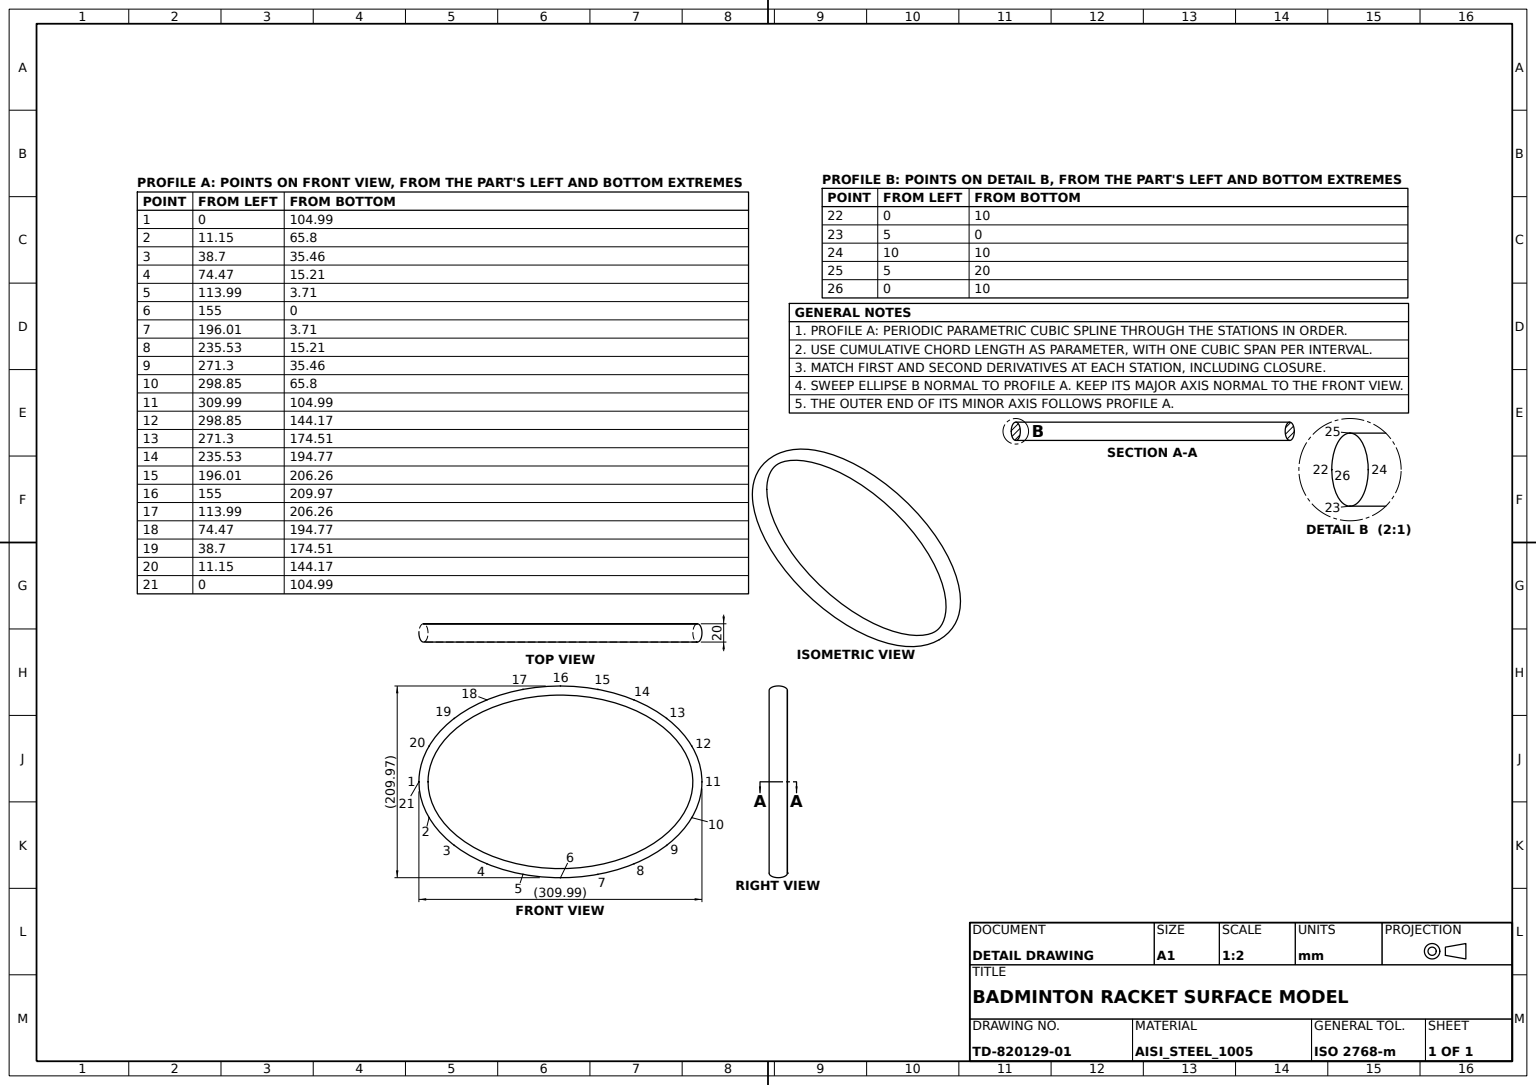
ISO-10303-21;
HEADER;
FILE_DESCRIPTION((''),'2;1');
FILE_NAME('','',(''),(''),'','','');
FILE_SCHEMA(('AUTOMOTIVE_DESIGN'));
ENDSEC;
DATA;
#1=APPLICATION_CONTEXT('');
#2=PRODUCT_CONTEXT('',#1,'mechanical');
#3=PRODUCT('','','',(#2));
#4=PRODUCT_DEFINITION_FORMATION('','',#3);
#5=PRODUCT_DEFINITION_CONTEXT('',#1,'design');
#6=PRODUCT_DEFINITION('','',#4,#5);
#7=PRODUCT_DEFINITION_SHAPE('','',#6);
#8=(LENGTH_UNIT()NAMED_UNIT(*)SI_UNIT(.MILLI.,.METRE.));
#9=(NAMED_UNIT(*)PLANE_ANGLE_UNIT()SI_UNIT($,.RADIAN.));
#10=(NAMED_UNIT(*)SI_UNIT($,.STERADIAN.)SOLID_ANGLE_UNIT());
#11=UNCERTAINTY_MEASURE_WITH_UNIT(LENGTH_MEASURE(0.005),#8,'distance_accuracy_value','');
#12=(GEOMETRIC_REPRESENTATION_CONTEXT(3)GLOBAL_UNCERTAINTY_ASSIGNED_CONTEXT((#11))GLOBAL_UNIT_ASSIGNED_CONTEXT((#8,#9,#10))REPRESENTATION_CONTEXT('',''));
#13=CARTESIAN_POINT('',(155.,0.,0.));
#14=VERTEX_POINT('',#13);
#15=VERTEX_LOOP('',#14);
#16=FACE_BOUND('',#15,.T.);
#17=CARTESIAN_POINT('',(155.,-4.365378,-3.535534));
#18=CARTESIAN_POINT('',(155.,4.365378,-3.535534));
#19=CARTESIAN_POINT('',(154.16152,13.313349,-3.535534));
#20=CARTESIAN_POINT('',(149.362746,30.331046,-3.535534));
#21=CARTESIAN_POINT('',(138.22226,49.513174,-3.535534));
#22=CARTESIAN_POINT('',(119.713466,67.928335,-3.535534));
#23=CARTESIAN_POINT('',(98.180606,82.120988,-3.535534));
#24=CARTESIAN_POINT('',(74.836894,92.619413,-3.535534));
#25=CARTESIAN_POINT('',(42.319091,102.226172,-3.535534));
#26=CARTESIAN_POINT('',(0.,106.826829,-3.535534));
#27=CARTESIAN_POINT('',(-42.31909,102.226172,-3.535534));
#28=CARTESIAN_POINT('',(-74.836894,92.619413,-3.535534));
#29=CARTESIAN_POINT('',(-98.180606,82.120988,-3.535534));
#30=CARTESIAN_POINT('',(-119.713466,67.928335,-3.535534));
#31=CARTESIAN_POINT('',(-138.22226,49.513174,-3.535534));
#32=CARTESIAN_POINT('',(-149.362746,30.331046,-3.535534));
#33=CARTESIAN_POINT('',(-154.161522,13.313342,-3.535534));
#34=CARTESIAN_POINT('',(-155.409023,0.000001,-3.535534));
#35=CARTESIAN_POINT('',(-154.161522,-13.313345,-3.535534));
#36=CARTESIAN_POINT('',(-149.362746,-30.331043,-3.535534));
#37=CARTESIAN_POINT('',(-138.22226,-49.513175,-3.535534));
#38=CARTESIAN_POINT('',(-119.713466,-67.928335,-3.535534));
#39=CARTESIAN_POINT('',(-98.180606,-82.120988,-3.535534));
#40=CARTESIAN_POINT('',(-74.836894,-92.619413,-3.535534));
#41=CARTESIAN_POINT('',(-42.319091,-102.226172,-3.535534));
#42=CARTESIAN_POINT('',(-0.000001,-106.82683,-3.535534));
#43=CARTESIAN_POINT('',(42.319096,-102.226171,-3.535534));
#44=CARTESIAN_POINT('',(74.836893,-92.619413,-3.535534));
#45=CARTESIAN_POINT('',(98.180607,-82.120988,-3.535534));
#46=CARTESIAN_POINT('',(119.713466,-67.928335,-3.535534));
#47=CARTESIAN_POINT('',(138.22226,-49.513174,-3.535534));
#48=CARTESIAN_POINT('',(149.362746,-30.331046,-3.535534));
#49=CARTESIAN_POINT('',(154.16152,-13.313349,-3.535534));
#50=CARTESIAN_POINT('',(155.,-4.365378,3.535534));
#51=CARTESIAN_POINT('',(155.,4.365378,3.535534));
#52=CARTESIAN_POINT('',(154.16152,13.313349,3.535534));
#53=CARTESIAN_POINT('',(149.362746,30.331046,3.535534));
#54=CARTESIAN_POINT('',(138.22226,49.513174,3.535534));
#55=CARTESIAN_POINT('',(119.713466,67.928335,3.535534));
#56=CARTESIAN_POINT('',(98.180606,82.120988,3.535534));
#57=CARTESIAN_POINT('',(74.836894,92.619413,3.535534));
#58=CARTESIAN_POINT('',(42.319091,102.226172,3.535534));
#59=CARTESIAN_POINT('',(0.,106.826829,3.535534));
#60=CARTESIAN_POINT('',(-42.31909,102.226172,3.535534));
#61=CARTESIAN_POINT('',(-74.836894,92.619413,3.535534));
#62=CARTESIAN_POINT('',(-98.180606,82.120988,3.535534));
#63=CARTESIAN_POINT('',(-119.713466,67.928335,3.535534));
#64=CARTESIAN_POINT('',(-138.22226,49.513174,3.535534));
#65=CARTESIAN_POINT('',(-149.362746,30.331046,3.535534));
#66=CARTESIAN_POINT('',(-154.161522,13.313342,3.535534));
#67=CARTESIAN_POINT('',(-155.409023,0.000001,3.535534));
#68=CARTESIAN_POINT('',(-154.161522,-13.313345,3.535534));
#69=CARTESIAN_POINT('',(-149.362746,-30.331043,3.535534));
#70=CARTESIAN_POINT('',(-138.22226,-49.513175,3.535534));
#71=CARTESIAN_POINT('',(-119.713466,-67.928335,3.535534));
#72=CARTESIAN_POINT('',(-98.180606,-82.120988,3.535534));
#73=CARTESIAN_POINT('',(-74.836894,-92.619413,3.535534));
#74=CARTESIAN_POINT('',(-42.319091,-102.226172,3.535534));
#75=CARTESIAN_POINT('',(-0.000001,-106.82683,3.535534));
#76=CARTESIAN_POINT('',(42.319096,-102.226171,3.535534));
#77=CARTESIAN_POINT('',(74.836893,-92.619413,3.535534));
#78=CARTESIAN_POINT('',(98.180607,-82.120988,3.535534));
#79=CARTESIAN_POINT('',(119.713466,-67.928335,3.535534));
#80=CARTESIAN_POINT('',(138.22226,-49.513174,3.535534));
#81=CARTESIAN_POINT('',(149.362746,-30.331046,3.535534));
#82=CARTESIAN_POINT('',(154.16152,-13.313349,3.535534));
#83=CARTESIAN_POINT('',(154.116117,-4.324056,8.232233));
#84=CARTESIAN_POINT('',(154.116117,4.324056,8.232233));
#85=CARTESIAN_POINT('',(153.288993,13.150839,8.232233));
#86=CARTESIAN_POINT('',(148.542341,29.983695,8.232233));
#87=CARTESIAN_POINT('',(137.516365,48.968656,8.232233));
#88=CARTESIAN_POINT('',(119.152954,67.239169,8.232233));
#89=CARTESIAN_POINT('',(97.753393,81.343963,8.232233));
#90=CARTESIAN_POINT('',(74.529005,91.788724,8.232233));
#91=CARTESIAN_POINT('',(42.144722,101.356037,8.232233));
#92=CARTESIAN_POINT('',(0.,105.937738,8.232233));
#93=CARTESIAN_POINT('',(-42.144721,101.356037,8.232233));
#94=CARTESIAN_POINT('',(-74.529005,91.788723,8.232233));
#95=CARTESIAN_POINT('',(-97.753393,81.343963,8.232233));
#96=CARTESIAN_POINT('',(-119.152954,67.239169,8.232233));
#97=CARTESIAN_POINT('',(-137.516365,48.968656,8.232233));
#98=CARTESIAN_POINT('',(-148.542341,29.983695,8.232233));
#99=CARTESIAN_POINT('',(-153.288994,13.150833,8.232233));
#100=CARTESIAN_POINT('',(-154.521268,0.000001,8.232233));
#101=CARTESIAN_POINT('',(-153.288994,-13.150836,8.232233));
#102=CARTESIAN_POINT('',(-148.542342,-29.983692,8.232233));
#103=CARTESIAN_POINT('',(-137.516364,-48.968657,8.232233));
#104=CARTESIAN_POINT('',(-119.152954,-67.239169,8.232233));
#105=CARTESIAN_POINT('',(-97.753393,-81.343963,8.232233));
#106=CARTESIAN_POINT('',(-74.529005,-91.788724,8.232233));
#107=CARTESIAN_POINT('',(-42.144722,-101.356037,8.232233));
#108=CARTESIAN_POINT('',(-0.000001,-105.937739,8.232233));
#109=CARTESIAN_POINT('',(42.144726,-101.356036,8.232233));
#110=CARTESIAN_POINT('',(74.529004,-91.788724,8.232233));
#111=CARTESIAN_POINT('',(97.753393,-81.343963,8.232233));
#112=CARTESIAN_POINT('',(119.152954,-67.239169,8.232233));
#113=CARTESIAN_POINT('',(137.516365,-48.968656,8.232233));
#114=CARTESIAN_POINT('',(148.542341,-29.983695,8.232233));
#115=CARTESIAN_POINT('',(153.288993,-13.150839,8.232233));
#116=CARTESIAN_POINT('',(151.767767,-4.214269,10.));
#117=CARTESIAN_POINT('',(151.767767,4.214269,10.));
#118=CARTESIAN_POINT('',(150.970814,12.719074,10.));
#119=CARTESIAN_POINT('',(146.362646,29.060832,10.));
#120=CARTESIAN_POINT('',(135.640904,47.521951,10.));
#121=CARTESIAN_POINT('',(117.663756,65.408156,10.));
#122=CARTESIAN_POINT('',(96.61835,79.27952,10.));
#123=CARTESIAN_POINT('',(73.710988,89.581704,10.));
#124=CARTESIAN_POINT('',(41.681448,99.044215,10.));
#125=CARTESIAN_POINT('',(0.,103.575552,10.));
#126=CARTESIAN_POINT('',(-41.681447,99.044216,10.));
#127=CARTESIAN_POINT('',(-73.710988,89.581704,10.));
#128=CARTESIAN_POINT('',(-96.61835,79.27952,10.));
#129=CARTESIAN_POINT('',(-117.663756,65.408156,10.));
#130=CARTESIAN_POINT('',(-135.640904,47.521951,10.));
#131=CARTESIAN_POINT('',(-146.362646,29.060832,10.));
#132=CARTESIAN_POINT('',(-150.970815,12.719071,10.));
#133=CARTESIAN_POINT('',(-152.162631,0.000001,10.));
#134=CARTESIAN_POINT('',(-150.970814,-12.719075,10.));
#135=CARTESIAN_POINT('',(-146.362647,-29.060829,10.));
#136=CARTESIAN_POINT('',(-135.640904,-47.521952,10.));
#137=CARTESIAN_POINT('',(-117.663756,-65.408156,10.));
#138=CARTESIAN_POINT('',(-96.61835,-79.27952,10.));
#139=CARTESIAN_POINT('',(-73.710988,-89.581704,10.));
#140=CARTESIAN_POINT('',(-41.681448,-99.044215,10.));
#141=CARTESIAN_POINT('',(-0.000001,-103.575553,10.));
#142=CARTESIAN_POINT('',(41.681452,-99.044214,10.));
#143=CARTESIAN_POINT('',(73.710987,-89.581704,10.));
#144=CARTESIAN_POINT('',(96.618351,-79.27952,10.));
#145=CARTESIAN_POINT('',(117.663756,-65.408156,10.));
#146=CARTESIAN_POINT('',(135.640904,-47.521951,10.));
#147=CARTESIAN_POINT('',(146.362646,-29.060832,10.));
#148=CARTESIAN_POINT('',(150.970814,-12.719074,10.));
#149=CARTESIAN_POINT('',(148.232233,-4.048981,10.));
#150=CARTESIAN_POINT('',(148.232233,4.048981,10.));
#151=CARTESIAN_POINT('',(147.480705,12.069035,10.));
#152=CARTESIAN_POINT('',(143.081029,27.671426,10.));
#153=CARTESIAN_POINT('',(132.817323,45.343879,10.));
#154=CARTESIAN_POINT('',(115.421709,62.651492,10.));
#155=CARTESIAN_POINT('',(94.909498,76.171419,10.));
#156=CARTESIAN_POINT('',(72.479431,86.258947,10.));
#157=CARTESIAN_POINT('',(40.98397,95.563675,10.));
#158=CARTESIAN_POINT('',(0.,100.019187,10.));
#159=CARTESIAN_POINT('',(-40.983969,95.563676,10.));
#160=CARTESIAN_POINT('',(-72.479431,86.258947,10.));
#161=CARTESIAN_POINT('',(-94.909498,76.171419,10.));
#162=CARTESIAN_POINT('',(-115.421709,62.651492,10.));
#163=CARTESIAN_POINT('',(-132.817323,45.343879,10.));
#164=CARTESIAN_POINT('',(-143.081029,27.671426,10.));
#165=CARTESIAN_POINT('',(-147.480704,12.069037,10.));
#166=CARTESIAN_POINT('',(-148.61161,0.000001,10.));
#167=CARTESIAN_POINT('',(-147.480703,-12.06904,10.));
#168=CARTESIAN_POINT('',(-143.081029,-27.671423,10.));
#169=CARTESIAN_POINT('',(-132.817322,-45.34388,10.));
#170=CARTESIAN_POINT('',(-115.421709,-62.651492,10.));
#171=CARTESIAN_POINT('',(-94.909498,-76.171419,10.));
#172=CARTESIAN_POINT('',(-72.479431,-86.258947,10.));
#173=CARTESIAN_POINT('',(-40.98397,-95.563675,10.));
#174=CARTESIAN_POINT('',(-0.000001,-100.019188,10.));
#175=CARTESIAN_POINT('',(40.983974,-95.563674,10.));
#176=CARTESIAN_POINT('',(72.47943,-86.258948,10.));
#177=CARTESIAN_POINT('',(94.909498,-76.171419,10.));
#178=CARTESIAN_POINT('',(115.421709,-62.651492,10.));
#179=CARTESIAN_POINT('',(132.817323,-45.343879,10.));
#180=CARTESIAN_POINT('',(143.081029,-27.671426,10.));
#181=CARTESIAN_POINT('',(147.480705,-12.069035,10.));
#182=CARTESIAN_POINT('',(145.883883,-3.939194,8.232233));
#183=CARTESIAN_POINT('',(145.883883,3.939194,8.232233));
#184=CARTESIAN_POINT('',(145.162526,11.63727,8.232233));
#185=CARTESIAN_POINT('',(140.901334,26.748563,8.232233));
#186=CARTESIAN_POINT('',(130.941862,43.897174,8.232233));
#187=CARTESIAN_POINT('',(113.932511,60.820478,8.232233));
#188=CARTESIAN_POINT('',(93.774455,74.106976,8.232233));
#189=CARTESIAN_POINT('',(71.661415,84.051927,8.232233));
#190=CARTESIAN_POINT('',(40.520696,93.251854,8.232233));
#191=CARTESIAN_POINT('',(0.,97.657001,8.232233));
#192=CARTESIAN_POINT('',(-40.520695,93.251854,8.232233));
#193=CARTESIAN_POINT('',(-71.661415,84.051927,8.232233));
#194=CARTESIAN_POINT('',(-93.774455,74.106976,8.232233));
#195=CARTESIAN_POINT('',(-113.932511,60.820478,8.232233));
#196=CARTESIAN_POINT('',(-130.941862,43.897174,8.232233));
#197=CARTESIAN_POINT('',(-140.901334,26.748563,8.232233));
#198=CARTESIAN_POINT('',(-145.162525,11.637276,8.232233));
#199=CARTESIAN_POINT('',(-146.252973,0.000001,8.232233));
#200=CARTESIAN_POINT('',(-145.162524,-11.637279,8.232233));
#201=CARTESIAN_POINT('',(-140.901334,-26.74856,8.232233));
#202=CARTESIAN_POINT('',(-130.941862,-43.897175,8.232233));
#203=CARTESIAN_POINT('',(-113.932511,-60.820478,8.232233));
#204=CARTESIAN_POINT('',(-93.774455,-74.106976,8.232233));
#205=CARTESIAN_POINT('',(-71.661415,-84.051927,8.232233));
#206=CARTESIAN_POINT('',(-40.520696,-93.251854,8.232233));
#207=CARTESIAN_POINT('',(-0.000001,-97.657002,8.232233));
#208=CARTESIAN_POINT('',(40.5207,-93.251853,8.232233));
#209=CARTESIAN_POINT('',(71.661413,-84.051928,8.232233));
#210=CARTESIAN_POINT('',(93.774455,-74.106976,8.232233));
#211=CARTESIAN_POINT('',(113.932511,-60.820478,8.232233));
#212=CARTESIAN_POINT('',(130.941862,-43.897174,8.232233));
#213=CARTESIAN_POINT('',(140.901334,-26.748563,8.232233));
#214=CARTESIAN_POINT('',(145.162526,-11.637269,8.232233));
#215=CARTESIAN_POINT('',(145.,-3.897872,3.535534));
#216=CARTESIAN_POINT('',(145.,3.897872,3.535534));
#217=CARTESIAN_POINT('',(144.289999,11.47476,3.535534));
#218=CARTESIAN_POINT('',(140.080929,26.401211,3.535534));
#219=CARTESIAN_POINT('',(130.235967,43.352656,3.535534));
#220=CARTESIAN_POINT('',(113.371999,60.131312,3.535534));
#221=CARTESIAN_POINT('',(93.347242,73.329951,3.535534));
#222=CARTESIAN_POINT('',(71.353525,83.221238,3.535534));
#223=CARTESIAN_POINT('',(40.346327,92.381719,3.535534));
#224=CARTESIAN_POINT('',(0.,96.76791,3.535534));
#225=CARTESIAN_POINT('',(-40.346326,92.381719,3.535534));
#226=CARTESIAN_POINT('',(-71.353525,83.221238,3.535534));
#227=CARTESIAN_POINT('',(-93.347242,73.329951,3.535534));
#228=CARTESIAN_POINT('',(-113.371999,60.131312,3.535534));
#229=CARTESIAN_POINT('',(-130.235967,43.352656,3.535534));
#230=CARTESIAN_POINT('',(-140.080929,26.401211,3.535534));
#231=CARTESIAN_POINT('',(-144.289997,11.474767,3.535534));
#232=CARTESIAN_POINT('',(-145.365218,0.000001,3.535534));
#233=CARTESIAN_POINT('',(-144.289996,-11.47477,3.535534));
#234=CARTESIAN_POINT('',(-140.08093,-26.401209,3.535534));
#235=CARTESIAN_POINT('',(-130.235966,-43.352657,3.535534));
#236=CARTESIAN_POINT('',(-113.371999,-60.131312,3.535534));
#237=CARTESIAN_POINT('',(-93.347242,-73.329951,3.535534));
#238=CARTESIAN_POINT('',(-71.353525,-83.221238,3.535534));
#239=CARTESIAN_POINT('',(-40.346327,-92.381719,3.535534));
#240=CARTESIAN_POINT('',(-0.000001,-96.76791,3.535534));
#241=CARTESIAN_POINT('',(40.346331,-92.381718,3.535534));
#242=CARTESIAN_POINT('',(71.353524,-83.221239,3.535534));
#243=CARTESIAN_POINT('',(93.347242,-73.329951,3.535534));
#244=CARTESIAN_POINT('',(113.371999,-60.131312,3.535534));
#245=CARTESIAN_POINT('',(130.235967,-43.352656,3.535534));
#246=CARTESIAN_POINT('',(140.080929,-26.401211,3.535534));
#247=CARTESIAN_POINT('',(144.289999,-11.47476,3.535534));
#248=CARTESIAN_POINT('',(145.,-3.897872,-3.535534));
#249=CARTESIAN_POINT('',(145.,3.897872,-3.535534));
#250=CARTESIAN_POINT('',(144.289999,11.47476,-3.535534));
#251=CARTESIAN_POINT('',(140.080929,26.401211,-3.535534));
#252=CARTESIAN_POINT('',(130.235967,43.352656,-3.535534));
#253=CARTESIAN_POINT('',(113.371999,60.131312,-3.535534));
#254=CARTESIAN_POINT('',(93.347242,73.329951,-3.535534));
#255=CARTESIAN_POINT('',(71.353525,83.221238,-3.535534));
#256=CARTESIAN_POINT('',(40.346327,92.381719,-3.535534));
#257=CARTESIAN_POINT('',(0.,96.76791,-3.535534));
#258=CARTESIAN_POINT('',(-40.346326,92.381719,-3.535534));
#259=CARTESIAN_POINT('',(-71.353525,83.221238,-3.535534));
#260=CARTESIAN_POINT('',(-93.347242,73.329951,-3.535534));
#261=CARTESIAN_POINT('',(-113.371999,60.131312,-3.535534));
#262=CARTESIAN_POINT('',(-130.235967,43.352656,-3.535534));
#263=CARTESIAN_POINT('',(-140.080929,26.401211,-3.535534));
#264=CARTESIAN_POINT('',(-144.289997,11.474767,-3.535534));
#265=CARTESIAN_POINT('',(-145.365218,0.000001,-3.535534));
#266=CARTESIAN_POINT('',(-144.289996,-11.47477,-3.535534));
#267=CARTESIAN_POINT('',(-140.08093,-26.401209,-3.535534));
#268=CARTESIAN_POINT('',(-130.235966,-43.352657,-3.535534));
#269=CARTESIAN_POINT('',(-113.371999,-60.131312,-3.535534));
#270=CARTESIAN_POINT('',(-93.347242,-73.329951,-3.535534));
#271=CARTESIAN_POINT('',(-71.353525,-83.221238,-3.535534));
#272=CARTESIAN_POINT('',(-40.346327,-92.381719,-3.535534));
#273=CARTESIAN_POINT('',(-0.000001,-96.76791,-3.535534));
#274=CARTESIAN_POINT('',(40.346331,-92.381718,-3.535534));
#275=CARTESIAN_POINT('',(71.353524,-83.221239,-3.535534));
#276=CARTESIAN_POINT('',(93.347242,-73.329951,-3.535534));
#277=CARTESIAN_POINT('',(113.371999,-60.131312,-3.535534));
#278=CARTESIAN_POINT('',(130.235967,-43.352656,-3.535534));
#279=CARTESIAN_POINT('',(140.080929,-26.401211,-3.535534));
#280=CARTESIAN_POINT('',(144.289999,-11.47476,-3.535534));
#281=CARTESIAN_POINT('',(145.883883,-3.939194,-8.232233));
#282=CARTESIAN_POINT('',(145.883883,3.939194,-8.232233));
#283=CARTESIAN_POINT('',(145.162526,11.63727,-8.232233));
#284=CARTESIAN_POINT('',(140.901334,26.748563,-8.232233));
#285=CARTESIAN_POINT('',(130.941862,43.897174,-8.232233));
#286=CARTESIAN_POINT('',(113.932511,60.820478,-8.232233));
#287=CARTESIAN_POINT('',(93.774455,74.106976,-8.232233));
#288=CARTESIAN_POINT('',(71.661415,84.051927,-8.232233));
#289=CARTESIAN_POINT('',(40.520696,93.251854,-8.232233));
#290=CARTESIAN_POINT('',(0.,97.657001,-8.232233));
#291=CARTESIAN_POINT('',(-40.520695,93.251854,-8.232233));
#292=CARTESIAN_POINT('',(-71.661415,84.051927,-8.232233));
#293=CARTESIAN_POINT('',(-93.774455,74.106976,-8.232233));
#294=CARTESIAN_POINT('',(-113.932511,60.820478,-8.232233));
#295=CARTESIAN_POINT('',(-130.941862,43.897174,-8.232233));
#296=CARTESIAN_POINT('',(-140.901334,26.748563,-8.232233));
#297=CARTESIAN_POINT('',(-145.162525,11.637276,-8.232233));
#298=CARTESIAN_POINT('',(-146.252973,0.000001,-8.232233));
#299=CARTESIAN_POINT('',(-145.162524,-11.637279,-8.232233));
#300=CARTESIAN_POINT('',(-140.901334,-26.74856,-8.232233));
#301=CARTESIAN_POINT('',(-130.941862,-43.897175,-8.232233));
#302=CARTESIAN_POINT('',(-113.932511,-60.820478,-8.232233));
#303=CARTESIAN_POINT('',(-93.774455,-74.106976,-8.232233));
#304=CARTESIAN_POINT('',(-71.661415,-84.051927,-8.232233));
#305=CARTESIAN_POINT('',(-40.520696,-93.251854,-8.232233));
#306=CARTESIAN_POINT('',(-0.000001,-97.657002,-8.232233));
#307=CARTESIAN_POINT('',(40.5207,-93.251853,-8.232233));
#308=CARTESIAN_POINT('',(71.661413,-84.051928,-8.232233));
#309=CARTESIAN_POINT('',(93.774455,-74.106976,-8.232233));
#310=CARTESIAN_POINT('',(113.932511,-60.820478,-8.232233));
#311=CARTESIAN_POINT('',(130.941862,-43.897174,-8.232233));
#312=CARTESIAN_POINT('',(140.901334,-26.748563,-8.232233));
#313=CARTESIAN_POINT('',(145.162526,-11.637269,-8.232233));
#314=CARTESIAN_POINT('',(148.232233,-4.048981,-10.));
#315=CARTESIAN_POINT('',(148.232233,4.048981,-10.));
#316=CARTESIAN_POINT('',(147.480705,12.069035,-10.));
#317=CARTESIAN_POINT('',(143.081029,27.671426,-10.));
#318=CARTESIAN_POINT('',(132.817323,45.343879,-10.));
#319=CARTESIAN_POINT('',(115.421709,62.651492,-10.));
#320=CARTESIAN_POINT('',(94.909498,76.171419,-10.));
#321=CARTESIAN_POINT('',(72.479431,86.258947,-10.));
#322=CARTESIAN_POINT('',(40.98397,95.563675,-10.));
#323=CARTESIAN_POINT('',(0.,100.019187,-10.));
#324=CARTESIAN_POINT('',(-40.983969,95.563676,-10.));
#325=CARTESIAN_POINT('',(-72.479431,86.258947,-10.));
#326=CARTESIAN_POINT('',(-94.909498,76.171419,-10.));
#327=CARTESIAN_POINT('',(-115.421709,62.651492,-10.));
#328=CARTESIAN_POINT('',(-132.817323,45.343879,-10.));
#329=CARTESIAN_POINT('',(-143.081029,27.671426,-10.));
#330=CARTESIAN_POINT('',(-147.480704,12.069037,-10.));
#331=CARTESIAN_POINT('',(-148.61161,0.000001,-10.));
#332=CARTESIAN_POINT('',(-147.480703,-12.06904,-10.));
#333=CARTESIAN_POINT('',(-143.081029,-27.671423,-10.));
#334=CARTESIAN_POINT('',(-132.817322,-45.34388,-10.));
#335=CARTESIAN_POINT('',(-115.421709,-62.651492,-10.));
#336=CARTESIAN_POINT('',(-94.909498,-76.171419,-10.));
#337=CARTESIAN_POINT('',(-72.479431,-86.258947,-10.));
#338=CARTESIAN_POINT('',(-40.98397,-95.563675,-10.));
#339=CARTESIAN_POINT('',(-0.000001,-100.019188,-10.));
#340=CARTESIAN_POINT('',(40.983974,-95.563674,-10.));
#341=CARTESIAN_POINT('',(72.47943,-86.258948,-10.));
#342=CARTESIAN_POINT('',(94.909498,-76.171419,-10.));
#343=CARTESIAN_POINT('',(115.421709,-62.651492,-10.));
#344=CARTESIAN_POINT('',(132.817323,-45.343879,-10.));
#345=CARTESIAN_POINT('',(143.081029,-27.671426,-10.));
#346=CARTESIAN_POINT('',(147.480705,-12.069035,-10.));
#347=CARTESIAN_POINT('',(151.767767,-4.214269,-10.));
#348=CARTESIAN_POINT('',(151.767767,4.214269,-10.));
#349=CARTESIAN_POINT('',(150.970814,12.719074,-10.));
#350=CARTESIAN_POINT('',(146.362646,29.060832,-10.));
#351=CARTESIAN_POINT('',(135.640904,47.521951,-10.));
#352=CARTESIAN_POINT('',(117.663756,65.408156,-10.));
#353=CARTESIAN_POINT('',(96.61835,79.27952,-10.));
#354=CARTESIAN_POINT('',(73.710988,89.581704,-10.));
#355=CARTESIAN_POINT('',(41.681448,99.044215,-10.));
#356=CARTESIAN_POINT('',(0.,103.575552,-10.));
#357=CARTESIAN_POINT('',(-41.681447,99.044216,-10.));
#358=CARTESIAN_POINT('',(-73.710988,89.581704,-10.));
#359=CARTESIAN_POINT('',(-96.61835,79.27952,-10.));
#360=CARTESIAN_POINT('',(-117.663756,65.408156,-10.));
#361=CARTESIAN_POINT('',(-135.640904,47.521951,-10.));
#362=CARTESIAN_POINT('',(-146.362646,29.060832,-10.));
#363=CARTESIAN_POINT('',(-150.970815,12.719071,-10.));
#364=CARTESIAN_POINT('',(-152.162631,0.000001,-10.));
#365=CARTESIAN_POINT('',(-150.970814,-12.719075,-10.));
#366=CARTESIAN_POINT('',(-146.362647,-29.060829,-10.));
#367=CARTESIAN_POINT('',(-135.640904,-47.521952,-10.));
#368=CARTESIAN_POINT('',(-117.663756,-65.408156,-10.));
#369=CARTESIAN_POINT('',(-96.61835,-79.27952,-10.));
#370=CARTESIAN_POINT('',(-73.710988,-89.581704,-10.));
#371=CARTESIAN_POINT('',(-41.681448,-99.044215,-10.));
#372=CARTESIAN_POINT('',(-0.000001,-103.575553,-10.));
#373=CARTESIAN_POINT('',(41.681452,-99.044214,-10.));
#374=CARTESIAN_POINT('',(73.710987,-89.581704,-10.));
#375=CARTESIAN_POINT('',(96.618351,-79.27952,-10.));
#376=CARTESIAN_POINT('',(117.663756,-65.408156,-10.));
#377=CARTESIAN_POINT('',(135.640904,-47.521951,-10.));
#378=CARTESIAN_POINT('',(146.362646,-29.060832,-10.));
#379=CARTESIAN_POINT('',(150.970814,-12.719074,-10.));
#380=CARTESIAN_POINT('',(154.116117,-4.324056,-8.232233));
#381=CARTESIAN_POINT('',(154.116117,4.324056,-8.232233));
#382=CARTESIAN_POINT('',(153.288993,13.150839,-8.232233));
#383=CARTESIAN_POINT('',(148.542341,29.983695,-8.232233));
#384=CARTESIAN_POINT('',(137.516365,48.968656,-8.232233));
#385=CARTESIAN_POINT('',(119.152954,67.239169,-8.232233));
#386=CARTESIAN_POINT('',(97.753393,81.343963,-8.232233));
#387=CARTESIAN_POINT('',(74.529005,91.788724,-8.232233));
#388=CARTESIAN_POINT('',(42.144722,101.356037,-8.232233));
#389=CARTESIAN_POINT('',(0.,105.937738,-8.232233));
#390=CARTESIAN_POINT('',(-42.144721,101.356037,-8.232233));
#391=CARTESIAN_POINT('',(-74.529005,91.788723,-8.232233));
#392=CARTESIAN_POINT('',(-97.753393,81.343963,-8.232233));
#393=CARTESIAN_POINT('',(-119.152954,67.239169,-8.232233));
#394=CARTESIAN_POINT('',(-137.516365,48.968656,-8.232233));
#395=CARTESIAN_POINT('',(-148.542341,29.983695,-8.232233));
#396=CARTESIAN_POINT('',(-153.288994,13.150833,-8.232233));
#397=CARTESIAN_POINT('',(-154.521268,0.000001,-8.232233));
#398=CARTESIAN_POINT('',(-153.288994,-13.150836,-8.232233));
#399=CARTESIAN_POINT('',(-148.542342,-29.983692,-8.232233));
#400=CARTESIAN_POINT('',(-137.516364,-48.968657,-8.232233));
#401=CARTESIAN_POINT('',(-119.152954,-67.239169,-8.232233));
#402=CARTESIAN_POINT('',(-97.753393,-81.343963,-8.232233));
#403=CARTESIAN_POINT('',(-74.529005,-91.788724,-8.232233));
#404=CARTESIAN_POINT('',(-42.144722,-101.356037,-8.232233));
#405=CARTESIAN_POINT('',(-0.000001,-105.937739,-8.232233));
#406=CARTESIAN_POINT('',(42.144726,-101.356036,-8.232233));
#407=CARTESIAN_POINT('',(74.529004,-91.788724,-8.232233));
#408=CARTESIAN_POINT('',(97.753393,-81.343963,-8.232233));
#409=CARTESIAN_POINT('',(119.152954,-67.239169,-8.232233));
#410=CARTESIAN_POINT('',(137.516365,-48.968656,-8.232233));
#411=CARTESIAN_POINT('',(148.542341,-29.983695,-8.232233));
#412=CARTESIAN_POINT('',(153.288993,-13.150839,-8.232233));
#413=(BOUNDED_SURFACE()B_SPLINE_SURFACE(4,3,((#17,#18,#19,#20,#21,#22,#23,#24,#25,#26,#27,#28,#29,#30,#31,#32,#33,#34,#35,#36,#37,#38,#39,#40,#41,#42,#43,#44,#45,#46,#47,#48,#49,#17,#18),(#50,#51,#52,#53,#54,#55,#56,#57,#58,#59,#60,#61,#62,#63,#64,#65,#66,#67,#68,#69,#70,#71,#72,#73,#74,#75,#76,#77,#78,#79,#80,#81,#82,#50,#51),(#83,#84,#85,#86,#87,#88,#89,#90,#91,#92,#93,#94,#95,#96,#97,#98,#99,#100,#101,#102,#103,#104,#105,#106,#107,#108,#109,#110,#111,#112,#113,#114,#115,#83,#84),(#116,#117,#118,#119,#120,#121,#122,#123,#124,#125,#126,#127,#128,#129,#130,#131,#132,#133,#134,#135,#136,#137,#138,#139,#140,#141,#142,#143,#144,#145,#146,#147,#148,#116,#117),(#149,#150,#151,#152,#153,#154,#155,#156,#157,#158,#159,#160,#161,#162,#163,#164,#165,#166,#167,#168,#169,#170,#171,#172,#173,#174,#175,#176,#177,#178,#179,#180,#181,#149,#150),(#182,#183,#184,#185,#186,#187,#188,#189,#190,#191,#192,#193,#194,#195,#196,#197,#198,#199,#200,#201,#202,#203,#204,#205,#206,#207,#208,#209,#210,#211,#212,#213,#214,#182,#183),(#215,#216,#217,#218,#219,#220,#221,#222,#223,#224,#225,#226,#227,#228,#229,#230,#231,#232,#233,#234,#235,#236,#237,#238,#239,#240,#241,#242,#243,#244,#245,#246,#247,#215,#216),(#248,#249,#250,#251,#252,#253,#254,#255,#256,#257,#258,#259,#260,#261,#262,#263,#264,#265,#266,#267,#268,#269,#270,#271,#272,#273,#274,#275,#276,#277,#278,#279,#280,#248,#249),(#281,#282,#283,#284,#285,#286,#287,#288,#289,#290,#291,#292,#293,#294,#295,#296,#297,#298,#299,#300,#301,#302,#303,#304,#305,#306,#307,#308,#309,#310,#311,#312,#313,#281,#282),(#314,#315,#316,#317,#318,#319,#320,#321,#322,#323,#324,#325,#326,#327,#328,#329,#330,#331,#332,#333,#334,#335,#336,#337,#338,#339,#340,#341,#342,#343,#344,#345,#346,#314,#315),(#347,#348,#349,#350,#351,#352,#353,#354,#355,#356,#357,#358,#359,#360,#361,#362,#363,#364,#365,#366,#367,#368,#369,#370,#371,#372,#373,#374,#375,#376,#377,#378,#379,#347,#348),(#380,#381,#382,#383,#384,#385,#386,#387,#388,#389,#390,#391,#392,#393,#394,#395,#396,#397,#398,#399,#400,#401,#402,#403,#404,#405,#406,#407,#408,#409,#410,#411,#412,#380,#381),(#17,#18,#19,#20,#21,#22,#23,#24,#25,#26,#27,#28,#29,#30,#31,#32,#33,#34,#35,#36,#37,#38,#39,#40,#41,#42,#43,#44,#45,#46,#47,#48,#49,#17,#18),(#50,#51,#52,#53,#54,#55,#56,#57,#58,#59,#60,#61,#62,#63,#64,#65,#66,#67,#68,#69,#70,#71,#72,#73,#74,#75,#76,#77,#78,#79,#80,#81,#82,#50,#51)),.UNSPECIFIED.,.T.,.T.,.F.)B_SPLINE_SURFACE_WITH_KNOTS((2,3,3,3,3,3,2),(1,1,2,1,1,1,1,1,1,1,1,1,1,1,1,1,1,1,1,1,1,1,1,1,1,1,1,1,1,1,1,1,1,1,2,1,1),(-0.25,0.,0.25,0.5,0.75,1.,1.25),(-0.03125,-0.015625,0.,0.015625,0.03125,0.0625,0.09375,0.125,0.15625,0.1875,0.25,0.3125,0.34375,0.375,0.40625,0.4375,0.46875,0.484375,0.5,0.515625,0.53125,0.5625,0.59375,0.625,0.65625,0.6875,0.75,0.8125,0.84375,0.875,0.90625,0.9375,0.96875,0.984375,1.,1.015625,1.03125),.UNSPECIFIED.)GEOMETRIC_REPRESENTATION_ITEM()RATIONAL_B_SPLINE_SURFACE(((0.585786438,0.585786438,0.585786438,0.585786438,0.585786438,0.585786438,0.585786438,0.585786438,0.585786438,0.585786438,0.585786438,0.585786438,0.585786438,0.585786438,0.585786438,0.585786438,0.585786438,0.585786438,0.585786438,0.585786438,0.585786438,0.585786438,0.585786438,0.585786438,0.585786438,0.585786438,0.585786438,0.585786438,0.585786438,0.585786438,0.585786438,0.585786438,0.585786438,0.585786438,0.585786438),(0.585786438,0.585786438,0.585786438,0.585786438,0.585786438,0.585786438,0.585786438,0.585786438,0.585786438,0.585786438,0.585786438,0.585786438,0.585786438,0.585786438,0.585786438,0.585786438,0.585786438,0.585786438,0.585786438,0.585786438,0.585786438,0.585786438,0.585786438,0.585786438,0.585786438,0.585786438,0.585786438,0.585786438,0.585786438,0.585786438,0.585786438,0.585786438,0.585786438,0.585786438,0.585786438),(0.55228475,0.55228475,0.55228475,0.55228475,0.55228475,0.55228475,0.55228475,0.55228475,0.55228475,0.55228475,0.55228475,0.55228475,0.55228475,0.55228475,0.55228475,0.55228475,0.55228475,0.55228475,0.55228475,0.55228475,0.55228475,0.55228475,0.55228475,0.55228475,0.55228475,0.55228475,0.55228475,0.55228475,0.55228475,0.55228475,0.55228475,0.55228475,0.55228475,0.55228475,0.55228475),(0.585786438,0.585786438,0.585786438,0.585786438,0.585786438,0.585786438,0.585786438,0.585786438,0.585786438,0.585786438,0.585786438,0.585786438,0.585786438,0.585786438,0.585786438,0.585786438,0.585786438,0.585786438,0.585786438,0.585786438,0.585786438,0.585786438,0.585786438,0.585786438,0.585786438,0.585786438,0.585786438,0.585786438,0.585786438,0.585786438,0.585786438,0.585786438,0.585786438,0.585786438,0.585786438),(0.585786438,0.585786438,0.585786438,0.585786438,0.585786438,0.585786438,0.585786438,0.585786438,0.585786438,0.585786438,0.585786438,0.585786438,0.585786438,0.585786438,0.585786438,0.585786438,0.585786438,0.585786438,0.585786438,0.585786438,0.585786438,0.585786438,0.585786438,0.585786438,0.585786438,0.585786438,0.585786438,0.585786438,0.585786438,0.585786438,0.585786438,0.585786438,0.585786438,0.585786438,0.585786438),(0.55228475,0.55228475,0.55228475,0.55228475,0.55228475,0.55228475,0.55228475,0.55228475,0.55228475,0.55228475,0.55228475,0.55228475,0.55228475,0.55228475,0.55228475,0.55228475,0.55228475,0.55228475,0.55228475,0.55228475,0.55228475,0.55228475,0.55228475,0.55228475,0.55228475,0.55228475,0.55228475,0.55228475,0.55228475,0.55228475,0.55228475,0.55228475,0.55228475,0.55228475,0.55228475),(0.585786438,0.585786438,0.585786438,0.585786438,0.585786438,0.585786438,0.585786438,0.585786438,0.585786438,0.585786438,0.585786438,0.585786438,0.585786438,0.585786438,0.585786438,0.585786438,0.585786438,0.585786438,0.585786438,0.585786438,0.585786438,0.585786438,0.585786438,0.585786438,0.585786438,0.585786438,0.585786438,0.585786438,0.585786438,0.585786438,0.585786438,0.585786438,0.585786438,0.585786438,0.585786438),(0.585786438,0.585786438,0.585786438,0.585786438,0.585786438,0.585786438,0.585786438,0.585786438,0.585786438,0.585786438,0.585786438,0.585786438,0.585786438,0.585786438,0.585786438,0.585786438,0.585786438,0.585786438,0.585786438,0.585786438,0.585786438,0.585786438,0.585786438,0.585786438,0.585786438,0.585786438,0.585786438,0.585786438,0.585786438,0.585786438,0.585786438,0.585786438,0.585786438,0.585786438,0.585786438),(0.55228475,0.55228475,0.55228475,0.55228475,0.55228475,0.55228475,0.55228475,0.55228475,0.55228475,0.55228475,0.55228475,0.55228475,0.55228475,0.55228475,0.55228475,0.55228475,0.55228475,0.55228475,0.55228475,0.55228475,0.55228475,0.55228475,0.55228475,0.55228475,0.55228475,0.55228475,0.55228475,0.55228475,0.55228475,0.55228475,0.55228475,0.55228475,0.55228475,0.55228475,0.55228475),(0.585786438,0.585786438,0.585786438,0.585786438,0.585786438,0.585786438,0.585786438,0.585786438,0.585786438,0.585786438,0.585786438,0.585786438,0.585786438,0.585786438,0.585786438,0.585786438,0.585786438,0.585786438,0.585786438,0.585786438,0.585786438,0.585786438,0.585786438,0.585786438,0.585786438,0.585786438,0.585786438,0.585786438,0.585786438,0.585786438,0.585786438,0.585786438,0.585786438,0.585786438,0.585786438),(0.585786438,0.585786438,0.585786438,0.585786438,0.585786438,0.585786438,0.585786438,0.585786438,0.585786438,0.585786438,0.585786438,0.585786438,0.585786438,0.585786438,0.585786438,0.585786438,0.585786438,0.585786438,0.585786438,0.585786438,0.585786438,0.585786438,0.585786438,0.585786438,0.585786438,0.585786438,0.585786438,0.585786438,0.585786438,0.585786438,0.585786438,0.585786438,0.585786438,0.585786438,0.585786438),(0.55228475,0.55228475,0.55228475,0.55228475,0.55228475,0.55228475,0.55228475,0.55228475,0.55228475,0.55228475,0.55228475,0.55228475,0.55228475,0.55228475,0.55228475,0.55228475,0.55228475,0.55228475,0.55228475,0.55228475,0.55228475,0.55228475,0.55228475,0.55228475,0.55228475,0.55228475,0.55228475,0.55228475,0.55228475,0.55228475,0.55228475,0.55228475,0.55228475,0.55228475,0.55228475),(0.585786438,0.585786438,0.585786438,0.585786438,0.585786438,0.585786438,0.585786438,0.585786438,0.585786438,0.585786438,0.585786438,0.585786438,0.585786438,0.585786438,0.585786438,0.585786438,0.585786438,0.585786438,0.585786438,0.585786438,0.585786438,0.585786438,0.585786438,0.585786438,0.585786438,0.585786438,0.585786438,0.585786438,0.585786438,0.585786438,0.585786438,0.585786438,0.585786438,0.585786438,0.585786438),(0.585786438,0.585786438,0.585786438,0.585786438,0.585786438,0.585786438,0.585786438,0.585786438,0.585786438,0.585786438,0.585786438,0.585786438,0.585786438,0.585786438,0.585786438,0.585786438,0.585786438,0.585786438,0.585786438,0.585786438,0.585786438,0.585786438,0.585786438,0.585786438,0.585786438,0.585786438,0.585786438,0.585786438,0.585786438,0.585786438,0.585786438,0.585786438,0.585786438,0.585786438,0.585786438)))REPRESENTATION_ITEM('')SURFACE());
#414=ADVANCED_FACE('',(#16),#413,.F.);
#415=CLOSED_SHELL('',(#414));
#416=MANIFOLD_SOLID_BREP('',#415);
#417=ADVANCED_BREP_SHAPE_REPRESENTATION('',(#416),#12);
#418=SHAPE_DEFINITION_REPRESENTATION(#7,#417);
ENDSEC;
END-ISO-10303-21;
